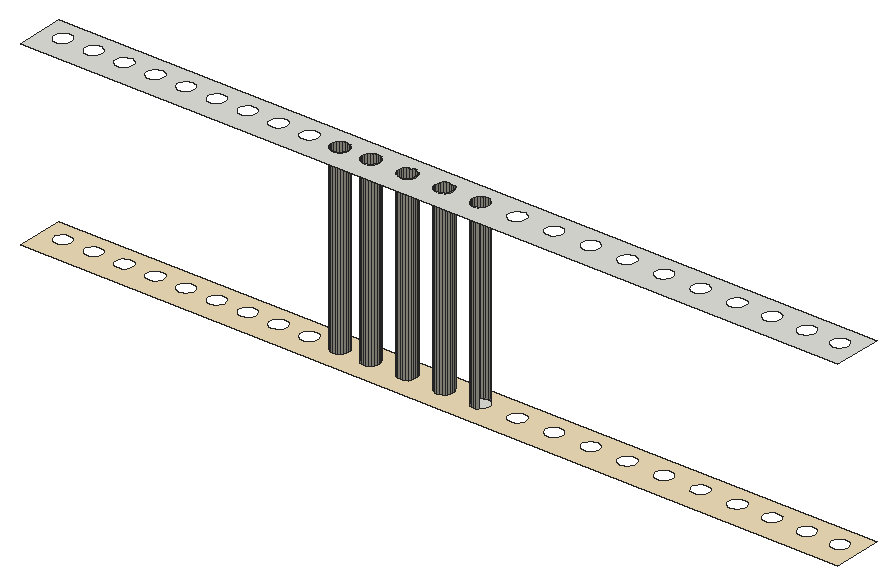
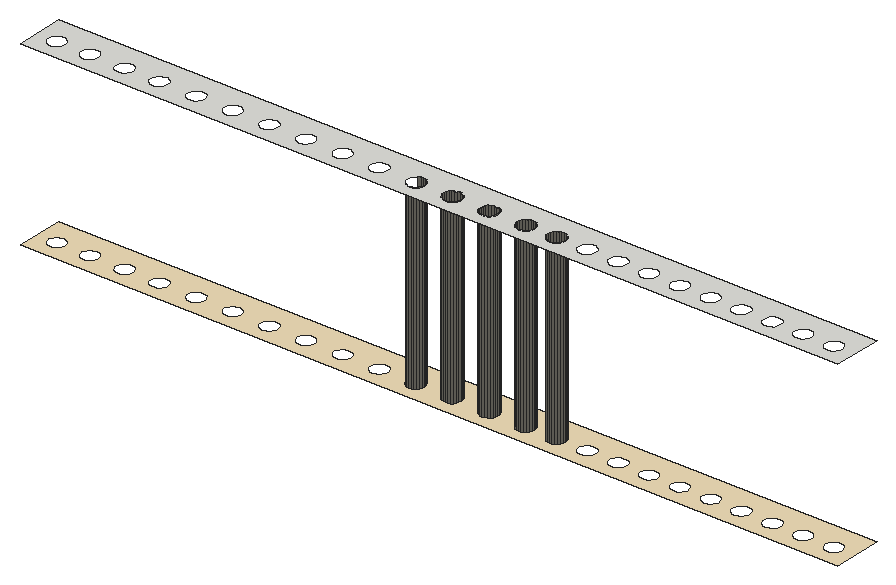
# SketchUp Ruby script. Lengths in inches.
U = 1.inch
M = Sketchup.active_model
def pt(a) = Geom::Point3d.new(a.map { |v| v * U })
def face(e, loops, mat)
  f = e.add_face(loops[0].map { |a| pt(a) })
  loops[1..].each { |l| e.add_face(l.map { |a| pt(a) }).erase! }
  f.material = f.back_material = mat if mat
  f
end
# faces: each face lists its corners as indices into pts; further lists are holes
def faces(e, pts, list, mat = nil) = list.each { |f| face(e, (f[0].is_a?(Array) ? f : [f]).map { |l| l.map { |i| pts[i] } }, mat) }
# xy, xz, yz: faces in a plane at the given z, y or x. An outline is a flat list of corners, or four numbers for a rectangle; further outlines are holes
def ring(l) = l.size == 4 ? [[l[0], l[1]], [l[2], l[1]], [l[2], l[3]], [l[0], l[3]]] : l.each_slice(2).to_a
def flat(e, list, mat, &to3) = list.each { |f| face(e, (f[0].is_a?(Array) ? f : [f]).map { |l| ring(l).map { |u, v| to3.(u, v) } }, mat) }
def xy(e, z, list, mat = nil) = flat(e, list, mat) { |x, y| [x, y, z] }
def xz(e, y, list, mat = nil) = flat(e, list, mat) { |x, z| [x, y, z] }
def yz(e, x, list, mat = nil) = flat(e, list, mat) { |y, z| [x, y, z] }
def lines(e, pts, list) = list.each { |a, b| e.add_line(pt(pts[a]), pt(pts[b])) }
# prism: a flat outline (further loops are holes) pulled along v
def prism(e, loops, v, mat = nil)
  f = face(e, loops, mat); d = Geom::Vector3d.new(v.map { |x| x * U })
  f.pushpull(f.normal.samedirection?(d) ? d.length : -d.length)
end
def box(e, o, s, mat = nil) = prism(e, [[o, [o[0] + s[0], o[1], o[2]], [o[0] + s[0], o[1] + s[1], o[2]], [o[0], o[1] + s[1], o[2]]]], [0, 0, s[2]], mat)
def at(x, y, z, deg = 0) = Geom::Transformation.translation(pt([x, y, z])) * Geom::Transformation.rotation(ORIGIN, Z_AXIS, deg.degrees)
def axes(o, x, y, z) = Geom::Transformation.new([*x, 0, *y, 0, *z, 0, *pt(o).to_a, 1])
def part(name) = M.definitions.add(name)
# library, detail: a bought-in or finely detailed component or shape, given as its bounding box
def library(name, o, s) = part(name).tap { |d| box(d.entities, o, s) }
def detail(e, o, s) = box(e.add_group.entities, o, s)
def put(e, d, t, mat = nil) = e.add_instance(d, t).tap { |i| i.material = mat if mat }
def group(e, t, mat = nil) = e.add_group.tap { |g| g.transformation = t; g.material = mat if mat }.entities
root = M.entities
M.materials.add("[Formica Graystone]").color = [149, 146, 135]
M.materials.add("[Quartz Light Brown]").color = [242, 223, 185]
xy(root,552.75,[[271.1875,21.93,270.48,22.02,269.8125,22.3,269.24,22.74,268.81,23.3,268.53,23.97,268.4375,24.68,268.53,25.39,268.81,26.05,269.24,26.625,269.8125,27.0625,270.48,27.34,271.1875,27.43,271.9,27.34,272.5625,27.0625,273.13,26.625,273.57,26.05,273.84,25.39,273.9375,24.68,273.84,23.97,273.57,23.3,273.13,22.74,272.5625,22.3,271.9,22.02],[280.75,21.93,280.04,22.02,279.375,22.3,278.81,22.74,278.37,23.3,278.09,23.97,278,24.68,278.09,25.39,278.37,26.05,278.81,26.625,279.375,27.0625,280.04,27.34,280.75,27.43,281.46,27.34,282.125,27.0625,282.69,26.625,283.13,26.05,283.41,25.39,283.5,24.68,283.41,23.97,283.13,23.3,282.69,22.74,282.125,22.3,281.46,22.02],[292.125,21.93,291.41,22.02,290.75,22.3,290.18,22.74,289.74,23.3,289.47,23.97,289.375,24.68,289.47,25.39,289.74,26.05,290.18,26.625,290.75,27.0625,291.41,27.34,292.125,27.43,292.84,27.34,293.5,27.0625,294.07,26.625,294.51,26.05,294.78,25.39,294.875,24.68,294.78,23.97,294.51,23.3,294.07,22.74,293.5,22.3,292.84,22.02],[303.5,21.93,302.79,22.02,302.125,22.3,301.56,22.74,301.12,23.3,300.84,23.97,300.75,24.68,300.84,25.39,301.12,26.05,301.56,26.625,302.125,27.0625,302.79,27.34,303.5,27.43,304.21,27.34,304.875,27.0625,305.44,26.625,305.88,26.05,306.16,25.39,306.25,24.68,306.16,23.97,305.88,23.3,305.44,22.74,304.875,22.3,304.21,22.02],[314.875,21.93,314.16,22.02,313.5,22.3,312.93,22.74,312.49,23.3,312.22,23.97,312.125,24.68,312.22,25.39,312.49,26.05,312.93,26.625,313.5,27.0625,314.16,27.34,314.875,27.43,315.59,27.34,316.25,27.0625,316.82,26.625,317.26,26.05,317.53,25.39,317.625,24.68,317.53,23.97,317.26,23.3,316.82,22.74,316.25,22.3,315.59,22.02]])
xy(root,552.75,[[[178.73,16.1875,432.54,31.11],[185.125,21.93,184.41,22.02,183.75,22.3,183.18,22.74,182.74,23.3,182.47,23.97,182.375,24.68,182.47,25.39,182.74,26.05,183.18,26.625,183.75,27.0625,184.41,27.34,185.125,27.43,185.84,27.34,186.5,27.0625,187.07,26.625,187.51,26.05,187.78,25.39,187.875,24.68,187.78,23.97,187.51,23.3,187.07,22.74,186.5,22.3,185.84,22.02],[194.6875,21.93,193.98,22.02,193.3125,22.3,192.74,22.74,192.31,23.3,192.03,23.97,191.9375,24.68,192.03,25.39,192.31,26.05,192.74,26.625,193.3125,27.0625,193.98,27.34,194.6875,27.43,195.4,27.34,196.0625,27.0625,196.63,26.625,197.07,26.05,197.34,25.39,197.4375,24.68,197.34,23.97,197.07,23.3,196.63,22.74,196.0625,22.3,195.4,22.02],[204.25,21.93,203.54,22.02,202.875,22.3,202.31,22.74,201.87,23.3,201.59,23.97,201.5,24.68,201.59,25.39,201.87,26.05,202.31,26.625,202.875,27.0625,203.54,27.34,204.25,27.43,204.96,27.34,205.625,27.0625,206.19,26.625,206.63,26.05,206.91,25.39,207,24.68,206.91,23.97,206.63,23.3,206.19,22.74,205.625,22.3,204.96,22.02],[213.8125,21.93,213.1,22.02,212.4375,22.3,211.87,22.74,211.43,23.3,211.16,23.97,211.0625,24.68,211.16,25.39,211.43,26.05,211.87,26.625,212.4375,27.0625,213.1,27.34,213.8125,27.43,214.52,27.34,215.1875,27.0625,215.76,26.625,216.19,26.05,216.47,25.39,216.5625,24.68,216.47,23.97,216.19,23.3,215.76,22.74,215.1875,22.3,214.52,22.02],[223.375,21.93,222.66,22.02,222,22.3,221.43,22.74,220.99,23.3,220.72,23.97,220.625,24.68,220.72,25.39,220.99,26.05,221.43,26.625,222,27.0625,222.66,27.34,223.375,27.43,224.09,27.34,224.75,27.0625,225.32,26.625,225.76,26.05,226.03,25.39,226.125,24.68,226.03,23.97,225.76,23.3,225.32,22.74,224.75,22.3,224.09,22.02],[232.9375,21.93,232.23,22.02,231.5625,22.3,230.99,22.74,230.56,23.3,230.28,23.97,230.1875,24.68,230.28,25.39,230.56,26.05,230.99,26.625,231.5625,27.0625,232.23,27.34,232.9375,27.43,233.65,27.34,234.3125,27.0625,234.88,26.625,235.32,26.05,235.59,25.39,235.6875,24.68,235.59,23.97,235.32,23.3,234.88,22.74,234.3125,22.3,233.65,22.02],[242.5,21.93,241.79,22.02,241.125,22.3,240.56,22.74,240.12,23.3,239.84,23.97,239.75,24.68,239.84,25.39,240.12,26.05,240.56,26.625,241.125,27.0625,241.79,27.34,242.5,27.43,243.21,27.34,243.875,27.0625,244.44,26.625,244.88,26.05,245.16,25.39,245.25,24.68,245.16,23.97,244.88,23.3,244.44,22.74,243.875,22.3,243.21,22.02],[252.0625,21.93,251.35,22.02,250.6875,22.3,250.12,22.74,249.68,23.3,249.41,23.97,249.3125,24.68,249.41,25.39,249.68,26.05,250.12,26.625,250.6875,27.0625,251.35,27.34,252.0625,27.43,252.77,27.34,253.4375,27.0625,254.01,26.625,254.44,26.05,254.72,25.39,254.8125,24.68,254.72,23.97,254.44,23.3,254.01,22.74,253.4375,22.3,252.77,22.02],[261.625,21.93,260.91,22.02,260.25,22.3,259.68,22.74,259.24,23.3,258.97,23.97,258.875,24.68,258.97,25.39,259.24,26.05,259.68,26.625,260.25,27.0625,260.91,27.34,261.625,27.43,262.34,27.34,263,27.0625,263.57,26.625,264.01,26.05,264.28,25.39,264.375,24.68,264.28,23.97,264.01,23.3,263.57,22.74,263,22.3,262.34,22.02],[271.1875,21.93,270.48,22.02,269.8125,22.3,269.24,22.74,268.81,23.3,268.53,23.97,268.4375,24.68,268.53,25.39,268.81,26.05,269.24,26.625,269.8125,27.0625,270.48,27.34,271.1875,27.43,271.9,27.34,272.5625,27.0625,273.13,26.625,273.57,26.05,273.84,25.39,273.9375,24.68,273.84,23.97,273.57,23.3,273.13,22.74,272.5625,22.3,271.9,22.02],[280.75,21.93,280.04,22.02,279.375,22.3,278.81,22.74,278.37,23.3,278.09,23.97,278,24.68,278.09,25.39,278.37,26.05,278.81,26.625,279.375,27.0625,280.04,27.34,280.75,27.43,281.46,27.34,282.125,27.0625,282.69,26.625,283.13,26.05,283.41,25.39,283.5,24.68,283.41,23.97,283.13,23.3,282.69,22.74,282.125,22.3,281.46,22.02],[292.125,21.93,291.41,22.02,290.75,22.3,290.18,22.74,289.74,23.3,289.47,23.97,289.375,24.68,289.47,25.39,289.74,26.05,290.18,26.625,290.75,27.0625,291.41,27.34,292.125,27.43,292.84,27.34,293.5,27.0625,294.07,26.625,294.51,26.05,294.78,25.39,294.875,24.68,294.78,23.97,294.51,23.3,294.07,22.74,293.5,22.3,292.84,22.02],[303.5,21.93,302.79,22.02,302.125,22.3,301.56,22.74,301.12,23.3,300.84,23.97,300.75,24.68,300.84,25.39,301.12,26.05,301.56,26.625,302.125,27.0625,302.79,27.34,303.5,27.43,304.21,27.34,304.875,27.0625,305.44,26.625,305.88,26.05,306.16,25.39,306.25,24.68,306.16,23.97,305.88,23.3,305.44,22.74,304.875,22.3,304.21,22.02],[314.875,21.93,314.16,22.02,313.5,22.3,312.93,22.74,312.49,23.3,312.22,23.97,312.125,24.68,312.22,25.39,312.49,26.05,312.93,26.625,313.5,27.0625,314.16,27.34,314.875,27.43,315.59,27.34,316.25,27.0625,316.82,26.625,317.26,26.05,317.53,25.39,317.625,24.68,317.53,23.97,317.26,23.3,316.82,22.74,316.25,22.3,315.59,22.02],[326.25,21.93,325.54,22.02,324.875,22.3,324.31,22.74,323.87,23.3,323.59,23.97,323.5,24.68,323.59,25.39,323.87,26.05,324.31,26.625,324.875,27.0625,325.54,27.34,326.25,27.43,326.96,27.34,327.625,27.0625,328.19,26.625,328.63,26.05,328.91,25.39,329,24.68,328.91,23.97,328.63,23.3,328.19,22.74,327.625,22.3,326.96,22.02],[337.625,21.93,336.91,22.02,336.25,22.3,335.68,22.74,335.24,23.3,334.97,23.97,334.875,24.68,334.97,25.39,335.24,26.05,335.68,26.625,336.25,27.0625,336.91,27.34,337.625,27.43,338.34,27.34,339,27.0625,339.57,26.625,340.01,26.05,340.28,25.39,340.375,24.68,340.28,23.97,340.01,23.3,339.57,22.74,339,22.3,338.34,22.02],[349,21.93,348.29,22.02,347.625,22.3,347.06,22.74,346.62,23.3,346.34,23.97,346.25,24.68,346.34,25.39,346.62,26.05,347.06,26.625,347.625,27.0625,348.29,27.34,349,27.43,349.71,27.34,350.375,27.0625,350.94,26.625,351.38,26.05,351.66,25.39,351.75,24.68,351.66,23.97,351.38,23.3,350.94,22.74,350.375,22.3,349.71,22.02],[360.375,21.93,359.66,22.02,359,22.3,358.43,22.74,357.99,23.3,357.72,23.97,357.625,24.68,357.72,25.39,357.99,26.05,358.43,26.625,359,27.0625,359.66,27.34,360.375,27.43,361.09,27.34,361.75,27.0625,362.32,26.625,362.76,26.05,363.03,25.39,363.125,24.68,363.03,23.97,362.76,23.3,362.32,22.74,361.75,22.3,361.09,22.02],[371.75,21.93,371.04,22.02,370.375,22.3,369.81,22.74,369.37,23.3,369.09,23.97,369,24.68,369.09,25.39,369.37,26.05,369.81,26.625,370.375,27.0625,371.04,27.34,371.75,27.43,372.46,27.34,373.125,27.0625,373.69,26.625,374.13,26.05,374.41,25.39,374.5,24.68,374.41,23.97,374.13,23.3,373.69,22.74,373.125,22.3,372.46,22.02],[383.125,21.93,382.41,22.02,381.75,22.3,381.18,22.74,380.74,23.3,380.47,23.97,380.375,24.68,380.47,25.39,380.74,26.05,381.18,26.625,381.75,27.0625,382.41,27.34,383.125,27.43,383.84,27.34,384.5,27.0625,385.07,26.625,385.51,26.05,385.78,25.39,385.875,24.68,385.78,23.97,385.51,23.3,385.07,22.74,384.5,22.3,383.84,22.02],[394.5,21.93,393.79,22.02,393.125,22.3,392.56,22.74,392.12,23.3,391.84,23.97,391.75,24.68,391.84,25.39,392.12,26.05,392.56,26.625,393.125,27.0625,393.79,27.34,394.5,27.43,395.21,27.34,395.875,27.0625,396.44,26.625,396.88,26.05,397.16,25.39,397.25,24.68,397.16,23.97,396.88,23.3,396.44,22.74,395.875,22.3,395.21,22.02],[426.375,21.93,425.66,22.02,425,22.3,424.43,22.74,423.99,23.3,423.72,23.97,423.625,24.68,423.72,25.39,423.99,26.05,424.43,26.625,425,27.0625,425.66,27.34,426.375,27.43,427.09,27.34,427.75,27.0625,428.32,26.625,428.76,26.05,429.03,25.39,429.125,24.68,429.03,23.97,428.76,23.3,428.32,22.74,427.75,22.3,427.09,22.02],[405.3125,21.93,404.6,22.02,403.9375,22.3,403.37,22.74,402.93,23.3,402.66,23.97,402.5625,24.68,402.66,25.39,402.93,26.05,403.37,26.625,403.9375,27.0625,404.6,27.34,405.3125,27.43,406.02,27.34,406.6875,27.0625,407.26,26.625,407.69,26.05,407.97,25.39,408.0625,24.68,407.97,23.97,407.69,23.3,407.26,22.74,406.6875,22.3,406.02,22.02],[416.125,21.93,415.41,22.02,414.75,22.3,414.18,22.74,413.74,23.3,413.47,23.97,413.375,24.68,413.47,25.39,413.74,26.05,414.18,26.625,414.75,27.0625,415.41,27.34,416.125,27.43,416.84,27.34,417.5,27.0625,418.07,26.625,418.51,26.05,418.78,25.39,418.875,24.68,418.78,23.97,418.51,23.3,418.07,22.74,417.5,22.3,416.84,22.02]]],"[Quartz Light Brown]")
xy(root,608.75,[[[178.73,16.1875,432.54,31.11],[185.125,21.93,185.84,22.02,186.5,22.3,187.07,22.74,187.51,23.3,187.78,23.97,187.875,24.68,187.78,25.39,187.51,26.05,187.07,26.625,186.5,27.0625,185.84,27.34,185.125,27.43,184.41,27.34,183.75,27.0625,183.18,26.625,182.74,26.05,182.47,25.39,182.375,24.68,182.47,23.97,182.74,23.3,183.18,22.74,183.75,22.3,184.41,22.02],[252.0625,21.93,252.77,22.02,253.4375,22.3,254.01,22.74,254.44,23.3,254.72,23.97,254.8125,24.68,254.72,25.39,254.44,26.05,254.01,26.625,253.4375,27.0625,252.77,27.34,252.0625,27.43,251.35,27.34,250.6875,27.0625,250.12,26.625,249.68,26.05,249.41,25.39,249.3125,24.68,249.41,23.97,249.68,23.3,250.12,22.74,250.6875,22.3,251.35,22.02],[371.75,21.93,372.46,22.02,373.125,22.3,373.69,22.74,374.13,23.3,374.41,23.97,374.5,24.68,374.41,25.39,374.13,26.05,373.69,26.625,373.125,27.0625,372.46,27.34,371.75,27.43,371.04,27.34,370.375,27.0625,369.81,26.625,369.37,26.05,369.09,25.39,369,24.68,369.09,23.97,369.37,23.3,369.81,22.74,370.375,22.3,371.04,22.02],[360.375,21.93,361.09,22.02,361.75,22.3,362.32,22.74,362.76,23.3,363.03,23.97,363.125,24.68,363.03,25.39,362.76,26.05,362.32,26.625,361.75,27.0625,361.09,27.34,360.375,27.43,359.66,27.34,359,27.0625,358.43,26.625,357.99,26.05,357.72,25.39,357.625,24.68,357.72,23.97,357.99,23.3,358.43,22.74,359,22.3,359.66,22.02],[303.5,21.93,304.21,22.02,304.875,22.3,305.44,22.74,305.88,23.3,306.16,23.97,306.25,24.68,306.16,25.39,305.88,26.05,305.44,26.625,304.875,27.0625,304.21,27.34,303.5,27.43,302.79,27.34,302.125,27.0625,301.56,26.625,301.12,26.05,300.84,25.39,300.75,24.68,300.84,23.97,301.12,23.3,301.56,22.74,302.125,22.3,302.79,22.02],[261.625,21.93,262.34,22.02,263,22.3,263.57,22.74,264.01,23.3,264.28,23.97,264.375,24.68,264.28,25.39,264.01,26.05,263.57,26.625,263,27.0625,262.34,27.34,261.625,27.43,260.91,27.34,260.25,27.0625,259.68,26.625,259.24,26.05,258.97,25.39,258.875,24.68,258.97,23.97,259.24,23.3,259.68,22.74,260.25,22.3,260.91,22.02],[242.5,21.93,243.21,22.02,243.875,22.3,244.44,22.74,244.88,23.3,245.16,23.97,245.25,24.68,245.16,25.39,244.88,26.05,244.44,26.625,243.875,27.0625,243.21,27.34,242.5,27.43,241.79,27.34,241.125,27.0625,240.56,26.625,240.12,26.05,239.84,25.39,239.75,24.68,239.84,23.97,240.12,23.3,240.56,22.74,241.125,22.3,241.79,22.02],[194.6875,21.93,195.4,22.02,196.0625,22.3,196.63,22.74,197.07,23.3,197.34,23.97,197.4375,24.68,197.34,25.39,197.07,26.05,196.63,26.625,196.0625,27.0625,195.4,27.34,194.6875,27.43,193.98,27.34,193.3125,27.0625,192.74,26.625,192.31,26.05,192.03,25.39,191.9375,24.68,192.03,23.97,192.31,23.3,192.74,22.74,193.3125,22.3,193.98,22.02],[383.125,21.93,383.84,22.02,384.5,22.3,385.07,22.74,385.51,23.3,385.78,23.97,385.875,24.68,385.78,25.39,385.51,26.05,385.07,26.625,384.5,27.0625,383.84,27.34,383.125,27.43,382.41,27.34,381.75,27.0625,381.18,26.625,380.74,26.05,380.47,25.39,380.375,24.68,380.47,23.97,380.74,23.3,381.18,22.74,381.75,22.3,382.41,22.02],[292.125,21.93,292.84,22.02,293.5,22.3,294.07,22.74,294.51,23.3,294.78,23.97,294.875,24.68,294.78,25.39,294.51,26.05,294.07,26.625,293.5,27.0625,292.84,27.34,292.125,27.43,291.41,27.34,290.75,27.0625,290.18,26.625,289.74,26.05,289.47,25.39,289.375,24.68,289.47,23.97,289.74,23.3,290.18,22.74,290.75,22.3,291.41,22.02],[271.1875,21.93,271.9,22.02,272.5625,22.3,273.13,22.74,273.57,23.3,273.84,23.97,273.9375,24.68,273.84,25.39,273.57,26.05,273.13,26.625,272.5625,27.0625,271.9,27.34,271.1875,27.43,270.48,27.34,269.8125,27.0625,269.24,26.625,268.81,26.05,268.53,25.39,268.4375,24.68,268.53,23.97,268.81,23.3,269.24,22.74,269.8125,22.3,270.48,22.02],[280.75,21.93,281.46,22.02,282.125,22.3,282.69,22.74,283.13,23.3,283.41,23.97,283.5,24.68,283.41,25.39,283.13,26.05,282.69,26.625,282.125,27.0625,281.46,27.34,280.75,27.43,280.04,27.34,279.375,27.0625,278.81,26.625,278.37,26.05,278.09,25.39,278,24.68,278.09,23.97,278.37,23.3,278.81,22.74,279.375,22.3,280.04,22.02],[223.375,21.93,224.09,22.02,224.75,22.3,225.32,22.74,225.76,23.3,226.03,23.97,226.125,24.68,226.03,25.39,225.76,26.05,225.32,26.625,224.75,27.0625,224.09,27.34,223.375,27.43,222.66,27.34,222,27.0625,221.43,26.625,220.99,26.05,220.72,25.39,220.625,24.68,220.72,23.97,220.99,23.3,221.43,22.74,222,22.3,222.66,22.02],[204.25,21.93,204.96,22.02,205.625,22.3,206.19,22.74,206.63,23.3,206.91,23.97,207,24.68,206.91,25.39,206.63,26.05,206.19,26.625,205.625,27.0625,204.96,27.34,204.25,27.43,203.54,27.34,202.875,27.0625,202.31,26.625,201.87,26.05,201.59,25.39,201.5,24.68,201.59,23.97,201.87,23.3,202.31,22.74,202.875,22.3,203.54,22.02],[416.125,21.93,416.84,22.02,417.5,22.3,418.07,22.74,418.51,23.3,418.78,23.97,418.875,24.68,418.78,25.39,418.51,26.05,418.07,26.625,417.5,27.0625,416.84,27.34,416.125,27.43,415.41,27.34,414.75,27.0625,414.18,26.625,413.74,26.05,413.47,25.39,413.375,24.68,413.47,23.97,413.74,23.3,414.18,22.74,414.75,22.3,415.41,22.02],[405.3125,21.93,406.02,22.02,406.6875,22.3,407.26,22.74,407.69,23.3,407.97,23.97,408.0625,24.68,407.97,25.39,407.69,26.05,407.26,26.625,406.6875,27.0625,406.02,27.34,405.3125,27.43,404.6,27.34,403.9375,27.0625,403.37,26.625,402.93,26.05,402.66,25.39,402.5625,24.68,402.66,23.97,402.93,23.3,403.37,22.74,403.9375,22.3,404.6,22.02],[314.875,21.93,315.59,22.02,316.25,22.3,316.82,22.74,317.26,23.3,317.53,23.97,317.625,24.68,317.53,25.39,317.26,26.05,316.82,26.625,316.25,27.0625,315.59,27.34,314.875,27.43,314.16,27.34,313.5,27.0625,312.93,26.625,312.49,26.05,312.22,25.39,312.125,24.68,312.22,23.97,312.49,23.3,312.93,22.74,313.5,22.3,314.16,22.02],[213.8125,21.93,214.52,22.02,215.1875,22.3,215.76,22.74,216.19,23.3,216.47,23.97,216.5625,24.68,216.47,25.39,216.19,26.05,215.76,26.625,215.1875,27.0625,214.52,27.34,213.8125,27.43,213.1,27.34,212.4375,27.0625,211.87,26.625,211.43,26.05,211.16,25.39,211.0625,24.68,211.16,23.97,211.43,23.3,211.87,22.74,212.4375,22.3,213.1,22.02],[349,21.93,349.71,22.02,350.375,22.3,350.94,22.74,351.38,23.3,351.66,23.97,351.75,24.68,351.66,25.39,351.38,26.05,350.94,26.625,350.375,27.0625,349.71,27.34,349,27.43,348.29,27.34,347.625,27.0625,347.06,26.625,346.62,26.05,346.34,25.39,346.25,24.68,346.34,23.97,346.62,23.3,347.06,22.74,347.625,22.3,348.29,22.02],[337.625,21.93,338.34,22.02,339,22.3,339.57,22.74,340.01,23.3,340.28,23.97,340.375,24.68,340.28,25.39,340.01,26.05,339.57,26.625,339,27.0625,338.34,27.34,337.625,27.43,336.91,27.34,336.25,27.0625,335.68,26.625,335.24,26.05,334.97,25.39,334.875,24.68,334.97,23.97,335.24,23.3,335.68,22.74,336.25,22.3,336.91,22.02],[326.25,21.93,326.96,22.02,327.625,22.3,328.19,22.74,328.63,23.3,328.91,23.97,329,24.68,328.91,25.39,328.63,26.05,328.19,26.625,327.625,27.0625,326.96,27.34,326.25,27.43,325.54,27.34,324.875,27.0625,324.31,26.625,323.87,26.05,323.59,25.39,323.5,24.68,323.59,23.97,323.87,23.3,324.31,22.74,324.875,22.3,325.54,22.02],[426.375,21.93,427.09,22.02,427.75,22.3,428.32,22.74,428.76,23.3,429.03,23.97,429.125,24.68,429.03,25.39,428.76,26.05,428.32,26.625,427.75,27.0625,427.09,27.34,426.375,27.43,425.66,27.34,425,27.0625,424.43,26.625,423.99,26.05,423.72,25.39,423.625,24.68,423.72,23.97,423.99,23.3,424.43,22.74,425,22.3,425.66,22.02],[394.5,21.93,395.21,22.02,395.875,22.3,396.44,22.74,396.88,23.3,397.16,23.97,397.25,24.68,397.16,25.39,396.88,26.05,396.44,26.625,395.875,27.0625,395.21,27.34,394.5,27.43,393.79,27.34,393.125,27.0625,392.56,26.625,392.12,26.05,391.84,25.39,391.75,24.68,391.84,23.97,392.12,23.3,392.56,22.74,393.125,22.3,393.79,22.02],[232.9375,21.93,233.65,22.02,234.3125,22.3,234.88,22.74,235.32,23.3,235.59,23.97,235.6875,24.68,235.59,25.39,235.32,26.05,234.88,26.625,234.3125,27.0625,233.65,27.34,232.9375,27.43,232.23,27.34,231.5625,27.0625,230.99,26.625,230.56,26.05,230.28,25.39,230.1875,24.68,230.28,23.97,230.56,23.3,230.99,22.74,231.5625,22.3,232.23,22.02]]])
p = [[270.48,22.02,552.75],[271.1875,21.93,552.75],[271.1875,21.93,608.75],[270.48,22.02,608.75],[271.9,22.02,552.75],[271.9,22.02,608.75],
  [280.04,22.02,552.75],[280.75,21.93,552.75],[280.75,21.93,608.75],[280.04,22.02,608.75],[281.46,22.02,552.75],[281.46,22.02,608.75],
  [291.41,22.02,552.75],[292.125,21.93,552.75],[292.125,21.93,608.75],[291.41,22.02,608.75],[292.84,22.02,552.75],[292.84,22.02,608.75],
  [302.79,22.02,552.75],[303.5,21.93,552.75],[303.5,21.93,608.75],[302.79,22.02,608.75],[304.21,22.02,552.75],[304.21,22.02,608.75],
  [314.16,22.02,552.75],[314.875,21.93,552.75],[314.875,21.93,608.75],[314.16,22.02,608.75],[315.59,22.02,552.75],[315.59,22.02,608.75],
  [269.8125,22.3,552.75],[269.8125,22.3,608.75],[272.5625,22.3,552.75],[272.5625,22.3,608.75],[279.375,22.3,552.75],[279.375,22.3,608.75],
  [282.125,22.3,552.75],[282.125,22.3,608.75],[290.75,22.3,552.75],[290.75,22.3,608.75],[293.5,22.3,552.75],[293.5,22.3,608.75],
  [302.125,22.3,552.75],[302.125,22.3,608.75],[304.875,22.3,552.75],[304.875,22.3,608.75],[313.5,22.3,552.75],[313.5,22.3,608.75],
  [316.25,22.3,552.75],[316.25,22.3,608.75],[269.24,22.74,552.75],[269.24,22.74,608.75],[273.13,22.74,552.75],[273.13,22.74,608.75],
  [278.81,22.74,552.75],[278.81,22.74,608.75],[282.69,22.74,552.75],[282.69,22.74,608.75],[290.18,22.74,552.75],[290.18,22.74,608.75],
  [294.07,22.74,552.75],[294.07,22.74,608.75],[301.56,22.74,552.75],[301.56,22.74,608.75],[305.44,22.74,552.75],[305.44,22.74,608.75],
  [312.93,22.74,552.75],[312.93,22.74,608.75],[268.81,23.3,552.75],[268.81,23.3,608.75],[273.57,23.3,552.75],[273.57,23.3,608.75],
  [278.37,23.3,552.75],[278.37,23.3,608.75],[283.13,23.3,552.75],[283.13,23.3,608.75],[289.74,23.3,552.75],[289.74,23.3,608.75],
  [294.51,23.3,552.75],[294.51,23.3,608.75],[301.12,23.3,552.75],[301.12,23.3,608.75],[305.88,23.3,552.75],[305.88,23.3,608.75],
  [312.49,23.3,552.75],[312.49,23.3,608.75],[268.53,23.97,552.75],[268.53,23.97,608.75],[273.84,23.97,552.75],[273.84,23.97,608.75],
  [278.09,23.97,552.75],[278.09,23.97,608.75],[283.41,23.97,552.75],[283.41,23.97,608.75],[289.47,23.97,552.75],[289.47,23.97,608.75],
  [294.78,23.97,552.75],[294.78,23.97,608.75],[300.84,23.97,552.75],[300.84,23.97,608.75],[306.16,23.97,552.75],[306.16,23.97,608.75],
  [312.22,23.97,552.75],[312.22,23.97,608.75],[268.4375,24.68,552.75],[268.4375,24.68,608.75],[273.9375,24.68,552.75],[273.9375,24.68,608.75],
  [278,24.68,552.75],[278,24.68,608.75],[283.5,24.68,552.75],[283.5,24.68,608.75],[289.375,24.68,552.75],[289.375,24.68,608.75],
  [294.875,24.68,552.75],[294.875,24.68,608.75],[300.75,24.68,552.75],[300.75,24.68,608.75],[306.25,24.68,552.75],[306.25,24.68,608.75],
  [312.125,24.68,552.75],[312.125,24.68,608.75],[268.53,25.39,552.75],[268.53,25.39,608.75],[273.84,25.39,552.75],[273.84,25.39,608.75],
  [278.09,25.39,552.75],[278.09,25.39,608.75],[283.41,25.39,552.75],[283.41,25.39,608.75],[289.47,25.39,552.75],[289.47,25.39,608.75],
  [294.78,25.39,552.75],[294.78,25.39,608.75],[300.84,25.39,552.75],[300.84,25.39,608.75],[306.16,25.39,552.75],[306.16,25.39,608.75],
  [312.22,25.39,552.75],[312.22,25.39,608.75],[268.81,26.05,552.75],[268.81,26.05,608.75],[273.57,26.05,552.75],[273.57,26.05,608.75],
  [278.37,26.05,552.75],[278.37,26.05,608.75],[283.13,26.05,552.75],[283.13,26.05,608.75],[289.74,26.05,552.75],[289.74,26.05,608.75],
  [294.51,26.05,552.75],[294.51,26.05,608.75],[301.12,26.05,552.75],[301.12,26.05,608.75],[305.88,26.05,552.75],[305.88,26.05,608.75],
  [312.49,26.05,552.75],[312.49,26.05,608.75],[269.24,26.625,552.75],[269.24,26.625,608.75],[273.13,26.625,552.75],[273.13,26.625,608.75],
  [278.81,26.625,552.75],[278.81,26.625,608.75],[282.69,26.625,552.75],[282.69,26.625,608.75],[290.18,26.625,552.75],[290.18,26.625,608.75],
  [294.07,26.625,552.75],[294.07,26.625,608.75],[301.56,26.625,552.75],[301.56,26.625,608.75],[305.44,26.625,552.75],[305.44,26.625,608.75],
  [312.93,26.625,552.75],[312.93,26.625,608.75],[269.8125,27.0625,552.75],[269.8125,27.0625,608.75],[272.5625,27.0625,552.75],[272.5625,27.0625,608.75],
  [279.375,27.0625,552.75],[279.375,27.0625,608.75],[282.125,27.0625,552.75],[282.125,27.0625,608.75],[290.75,27.0625,552.75],[290.75,27.0625,608.75],
  [293.5,27.0625,552.75],[293.5,27.0625,608.75],[302.125,27.0625,552.75],[302.125,27.0625,608.75],[304.875,27.0625,552.75],[304.875,27.0625,608.75],
  [313.5,27.0625,552.75],[313.5,27.0625,608.75],[270.48,27.34,552.75],[270.48,27.34,608.75],[271.9,27.34,552.75],[271.9,27.34,608.75],
  [280.04,27.34,552.75],[280.04,27.34,608.75],[281.46,27.34,552.75],[281.46,27.34,608.75],[291.41,27.34,552.75],[291.41,27.34,608.75],
  [292.84,27.34,552.75],[292.84,27.34,608.75],[302.79,27.34,552.75],[302.79,27.34,608.75],[304.21,27.34,552.75],[304.21,27.34,608.75],
  [314.16,27.34,552.75],[314.16,27.34,608.75],[316.25,27.0625,552.75],[315.59,27.34,552.75],[315.59,27.34,608.75],[316.25,27.0625,608.75],
  [271.1875,27.43,552.75],[271.1875,27.43,608.75],[280.75,27.43,552.75],[280.75,27.43,608.75],[292.125,27.43,552.75],[292.125,27.43,608.75],
  [303.5,27.43,552.75],[303.5,27.43,608.75],[314.875,27.43,552.75],[314.875,27.43,608.75]]
faces(root,p,[[0,1,2,3],[1,4,5,2],[6,7,8,9],[7,10,11,8],[12,13,14,15],[13,16,17,14],[18,19,20,21],[19,22,23,20],
  [24,25,26,27],[25,28,29,26],[30,0,3,31],[4,32,33,5],[34,6,9,35],[10,36,37,11],[38,12,15,39],[16,40,41,17],
  [42,18,21,43],[22,44,45,23],[46,24,27,47],[28,48,49,29],[50,30,31,51],[32,52,53,33],[54,34,35,55],[36,56,57,37],
  [58,38,39,59],[40,60,61,41],[62,42,43,63],[44,64,65,45],[66,46,47,67],[68,50,51,69],[52,70,71,53],[72,54,55,73],
  [56,74,75,57],[76,58,59,77],[60,78,79,61],[80,62,63,81],[64,82,83,65],[84,66,67,85],[86,68,69,87],[70,88,89,71],
  [90,72,73,91],[74,92,93,75],[94,76,77,95],[78,96,97,79],[98,80,81,99],[82,100,101,83],[102,84,85,103],[104,86,87,105],
  [88,106,107,89],[108,90,91,109],[92,110,111,93],[112,94,95,113],[96,114,115,97],[116,98,99,117],[100,118,119,101],[120,102,103,121],
  [122,104,105,123],[106,124,125,107],[126,108,109,127],[110,128,129,111],[130,112,113,131],[114,132,133,115],[134,116,117,135],[118,136,137,119],
  [138,120,121,139],[140,122,123,141],[124,142,143,125],[144,126,127,145],[128,146,147,129],[148,130,131,149],[132,150,151,133],[152,134,135,153],
  [136,154,155,137],[156,138,139,157],[158,140,141,159],[142,160,161,143],[162,144,145,163],[146,164,165,147],[166,148,149,167],[150,168,169,151],
  [170,152,153,171],[154,172,173,155],[174,156,157,175],[176,158,159,177],[160,178,179,161],[180,162,163,181],[164,182,183,165],[184,166,167,185],
  [168,186,187,169],[188,170,171,189],[172,190,191,173],[192,174,175,193],[194,176,177,195],[178,196,197,179],[198,180,181,199],[182,200,201,183],
  [202,184,185,203],[186,204,205,187],[206,188,189,207],[190,208,209,191],[210,192,193,211],[212,213,214,215],[216,194,195,217],[196,216,217,197],
  [218,198,199,219],[200,218,219,201],[220,202,203,221],[204,220,221,205],[222,206,207,223],[208,222,223,209],[224,210,211,225],[213,224,225,214]],"[Formica Graystone]")
